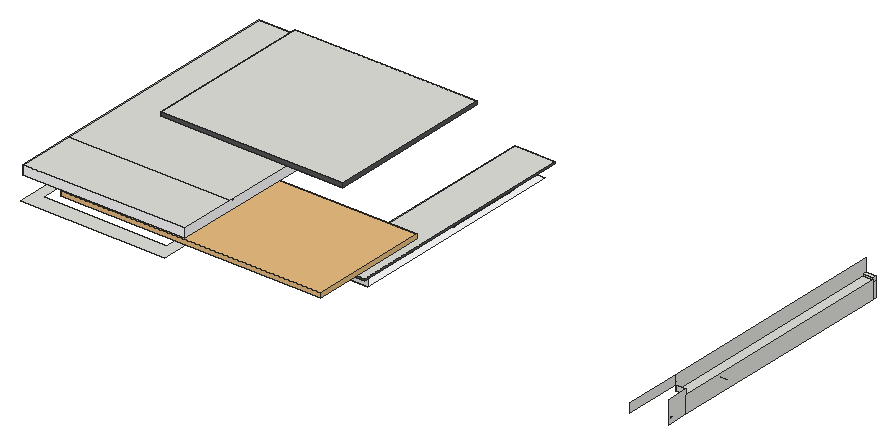
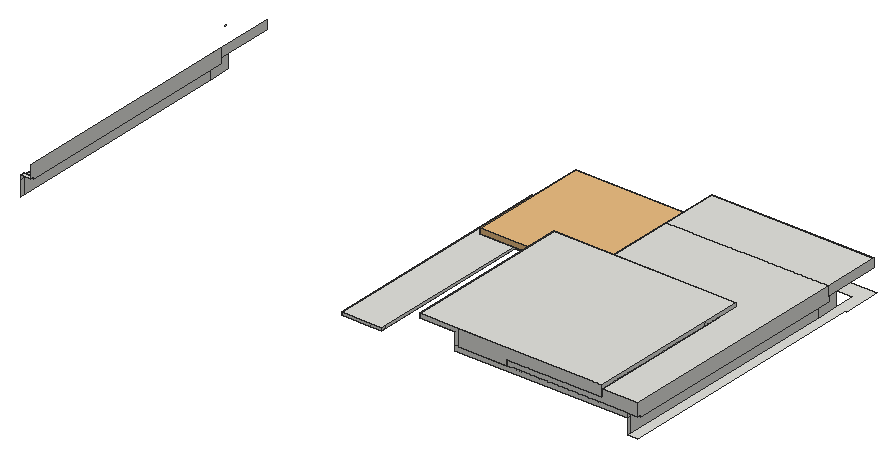
# SketchUp Ruby script. Lengths in inches.
U = 1.inch
M = Sketchup.active_model
def pt(a) = Geom::Point3d.new(a.map { |v| v * U })
def face(e, loops, mat)
  f = e.add_face(loops[0].map { |a| pt(a) })
  loops[1..].each { |l| e.add_face(l.map { |a| pt(a) }).erase! }
  f.material = f.back_material = mat if mat
  f
end
# faces: each face lists its corners as indices into pts; further lists are holes
def faces(e, pts, list, mat = nil) = list.each { |f| face(e, (f[0].is_a?(Array) ? f : [f]).map { |l| l.map { |i| pts[i] } }, mat) }
# xy, xz, yz: faces in a plane at the given z, y or x. An outline is a flat list of corners, or four numbers for a rectangle; further outlines are holes
def ring(l) = l.size == 4 ? [[l[0], l[1]], [l[2], l[1]], [l[2], l[3]], [l[0], l[3]]] : l.each_slice(2).to_a
def flat(e, list, mat, &to3) = list.each { |f| face(e, (f[0].is_a?(Array) ? f : [f]).map { |l| ring(l).map { |u, v| to3.(u, v) } }, mat) }
def xy(e, z, list, mat = nil) = flat(e, list, mat) { |x, y| [x, y, z] }
def xz(e, y, list, mat = nil) = flat(e, list, mat) { |x, z| [x, y, z] }
def yz(e, x, list, mat = nil) = flat(e, list, mat) { |y, z| [x, y, z] }
def lines(e, pts, list) = list.each { |a, b| e.add_line(pt(pts[a]), pt(pts[b])) }
# prism: a flat outline (further loops are holes) pulled along v
def prism(e, loops, v, mat = nil)
  f = face(e, loops, mat); d = Geom::Vector3d.new(v.map { |x| x * U })
  f.pushpull(f.normal.samedirection?(d) ? d.length : -d.length)
end
def box(e, o, s, mat = nil) = prism(e, [[o, [o[0] + s[0], o[1], o[2]], [o[0] + s[0], o[1] + s[1], o[2]], [o[0], o[1] + s[1], o[2]]]], [0, 0, s[2]], mat)
def at(x, y, z, deg = 0) = Geom::Transformation.translation(pt([x, y, z])) * Geom::Transformation.rotation(ORIGIN, Z_AXIS, deg.degrees)
def axes(o, x, y, z) = Geom::Transformation.new([*x, 0, *y, 0, *z, 0, *pt(o).to_a, 1])
def part(name) = M.definitions.add(name)
# library, detail: a bought-in or finely detailed component or shape, given as its bounding box
def library(name, o, s) = part(name).tap { |d| box(d.entities, o, s) }
def detail(e, o, s) = box(e.add_group.entities, o, s)
def put(e, d, t, mat = nil) = e.add_instance(d, t).tap { |i| i.material = mat if mat }
def group(e, t, mat = nil) = e.add_group.tap { |g| g.transformation = t; g.material = mat if mat }.entities
root = M.entities
M.materials.add("[Color M00]").color = [255, 255, 255]
M.materials.add("[Color M06]").color = [86, 86, 86]
c1 = library("Mesh Light\#4",[-0.5,-0.5,-0.1],[1,1,0.2])
c2 = part("Group\#24")
xy(c2.entities,0,[[203.13,95.41,201.58,95.62,200.13,96.22,198.89,97.17,197.9375,98.41,197.34,99.86,197.13,101.41,197.34,102.96,197.9375,104.41,198.89,105.65,200.13,106.61,201.58,107.21,203.13,107.41,204.6875,107.21,206.13,106.61,207.375,105.65,208.33,104.41,208.93,102.96,209.13,101.41,208.93,99.86,208.33,98.41,207.375,97.17,206.13,96.22,204.6875,95.62],[281.57,95.41,280.02,95.62,278.57,96.22,277.33,97.17,276.375,98.41,275.77,99.86,275.57,101.41,275.77,102.96,276.375,104.41,277.33,105.65,278.57,106.61,280.02,107.21,281.57,107.41,283.125,107.21,284.57,106.61,285.8125,105.65,286.77,104.41,287.37,102.96,287.57,101.41,287.37,99.86,286.77,98.41,285.8125,97.17,284.57,96.22,283.125,95.62],[350.95,95.41,349.39,95.62,347.95,96.22,346.7,97.17,345.75,98.41,345.15,99.86,344.95,101.41,345.15,102.96,345.75,104.41,346.7,105.65,347.95,106.61,349.39,107.21,350.95,107.41,352.5,107.21,353.95,106.61,355.1875,105.65,356.14,104.41,356.74,102.96,356.95,101.41,356.74,99.86,356.14,98.41,355.1875,97.17,353.95,96.22,352.5,95.62],[376,162.85,374.44,163.05,373,163.65,371.75,164.6,370.8,165.85,370.2,167.29,370,168.85,370.2,170.4,370.8,171.85,371.75,173.09,373,174.04,374.44,174.64,376,174.85,377.55,174.64,379,174.04,380.24,173.09,381.19,171.85,381.79,170.4,382,168.85,381.79,167.29,381.19,165.85,380.24,164.6,379,163.65,377.55,163.05]],"[Color M00]")
xy(c2.entities,33.4375,[[6,0,4.45,0.2,3,0.8,1.76,1.76,0.8,3,0.2,4.45,0,6,0.2,7.55,0.8,9,1.76,10.24,3,11.2,4.45,11.8,6,12,7.55,11.8,9,11.2,10.24,10.24,11.2,9,11.8,7.55,12,6,11.8,4.45,11.2,3,10.24,1.76,9,0.8,7.55,0.2],[83.125,0,81.57,0.2,80.125,0.8,78.88,1.76,77.93,3,77.33,4.45,77.125,6,77.33,7.55,77.93,9,78.88,10.24,80.125,11.2,81.57,11.8,83.125,12,84.68,11.8,86.125,11.2,87.37,10.24,88.32,9,88.92,7.55,89.125,6,88.92,4.45,88.32,3,87.37,1.76,86.125,0.8,84.68,0.2],[166.6875,0,165.13,0.2,163.6875,0.8,162.44,1.76,161.49,3,160.89,4.45,160.6875,6,160.89,7.55,161.49,9,162.44,10.24,163.6875,11.2,165.13,11.8,166.6875,12,168.24,11.8,169.6875,11.2,170.93,10.24,171.88,9,172.48,7.55,172.6875,6,172.48,4.45,171.88,3,170.93,1.76,169.6875,0.8,168.24,0.2],[166.6875,88.9375,165.13,89.14,163.6875,89.74,162.44,90.69,161.49,91.9375,160.89,93.38,160.6875,94.9375,160.89,96.49,161.49,97.9375,162.44,99.18,163.6875,100.13,165.13,100.73,166.6875,100.9375,168.24,100.73,169.6875,100.13,170.93,99.18,171.88,97.9375,172.48,96.49,172.6875,94.9375,172.48,93.38,171.88,91.9375,170.93,90.69,169.6875,89.74,168.24,89.14]],"[Color M00]")
put(c2.entities,c1,axes([191,87.42,16.72],[382.99758,0,0],[0,175.84579,0],[0,0,34.4375]))
c3 = library("Group\#23",[-0.5,-0.5,-0.1],[13,110.375,0.2])
xy(root,269.375,[[278.36,584.06,490.8,584.06,490.8,676.67,484.3,676.67,484.3,706.17,475.29,706.17,475.29,607.33,294.47,607.33,294.47,1021.31,279.74,1021.31,279.74,638.99,278.36,638.99],[484.3,676.67,490.8,731.24]])
xy(root,269.375,[[[490.8,676.67,490.8,731.24,674.49,731.24,674.49,1001.66,715.11,1001.66,715.11,676.67],[604.45,698.72,606.01,698.92,607.45,699.52,608.7,700.47,609.65,701.72,610.25,703.16,610.45,704.72,610.25,706.27,609.65,707.72,608.7,708.96,607.45,709.91,606.01,710.51,604.45,710.72,602.9,710.51,601.45,709.91,600.21,708.96,599.26,707.72,598.66,706.27,598.45,704.72,598.66,703.16,599.26,701.72,600.21,700.47,601.45,699.52,602.9,698.92],[673.83,698.72,675.38,698.92,676.83,699.52,678.07,700.47,679.02,701.72,679.625,703.16,679.83,704.72,679.625,706.27,679.02,707.72,678.07,708.96,676.83,709.91,675.38,710.51,673.83,710.72,672.27,710.51,670.83,709.91,669.59,708.96,668.63,707.72,668.03,706.27,667.83,704.72,668.03,703.16,668.63,701.72,669.59,700.47,670.83,699.52,672.27,698.92],[526.02,698.72,527.57,698.92,529.02,699.52,530.26,700.47,531.21,701.72,531.8125,703.16,532.02,704.72,531.8125,706.27,531.21,707.72,530.26,708.96,529.02,709.91,527.57,710.51,526.02,710.72,524.46,710.51,523.02,709.91,521.77,708.96,520.82,707.72,520.22,706.27,520.02,704.72,520.22,703.16,520.82,701.72,521.77,700.47,523.02,699.52,524.46,698.92],[698.88,766.15,700.43,766.35,701.88,766.95,703.12,767.91,704.08,769.15,704.68,770.6,704.88,772.15,704.68,773.7,704.08,775.15,703.12,776.39,701.88,777.35,700.43,777.95,698.88,778.15,697.33,777.95,695.88,777.35,694.64,776.39,693.68,775.15,693.08,773.7,692.88,772.15,693.08,770.6,693.68,769.15,694.64,767.91,695.88,766.95,697.33,766.35],[698.88,846.59,700.43,846.79,701.88,847.39,703.12,848.35,704.08,849.59,704.68,851.04,704.88,852.59,704.68,854.14,704.08,855.59,703.12,856.83,701.88,857.78,700.43,858.38,698.88,858.59,697.33,858.38,695.88,857.78,694.64,856.83,693.68,855.59,693.08,854.14,692.88,852.59,693.08,851.04,693.68,849.59,694.64,848.35,695.88,847.39,697.33,846.79],[698.88,943.96,700.43,944.17,701.88,944.77,703.12,945.72,704.08,946.96,704.68,948.41,704.88,949.96,704.68,951.52,704.08,952.96,703.12,954.21,701.88,955.16,700.43,955.76,698.88,955.96,697.33,955.76,695.88,955.16,694.64,954.21,693.68,952.96,693.08,951.52,692.88,949.96,693.08,948.41,693.68,946.96,694.64,945.72,695.88,944.77,697.33,944.17]]],"[Color M00]")
xy(root,279.25,[[484.3,670.42,715.11,676.67],[484.3,676.67,484.3,776.62,655.66,776.62,655.66,1021.31,715.11,1021.31,715.11,676.67]])
xy(root,282.6875,[[484.3,670.42,715.11,670.42,715.11,1021.31,655.66,1021.31,655.66,776.62,484.3,776.62]])
xy(root,291.125,[[304.78,733.75,304.78,1014.93,471.68,1014.93,471.68,854.49,462.15,854.49,462.15,733.75],[471.68,854.49,542.11,1014.93]])
xy(root,294.9375,[[279.74,670.48,294.47,1014.93],[1172.33,670.48,1187.0625,1014.93]])
xy(root,297.875,[[279.74,1014.93,294.47,1021.31],[294.47,1014.93,471.68,1021.31],[471.68,1014.93,542.11,1021.31],[1172.33,1014.93,1187.0625,1021.31]])
xy(root,302.8125,[[[279.74,587.17,279.74,670.48,294.47,670.48,294.47,639.17,471.68,639.17,471.68,832.12,518.11,832.12,518.11,587.17],[328.88,603.3,330.44,603.51,331.88,604.11,333.125,605.0625,334.08,606.3,334.68,607.75,334.88,609.3,334.68,610.86,334.08,612.3,333.125,613.55,331.88,614.5,330.44,615.1,328.88,615.3,327.33,615.1,325.88,614.5,324.64,613.55,323.6875,612.3,323.09,610.86,322.88,609.3,323.09,607.75,323.6875,606.3,324.64,605.0625,325.88,604.11,327.33,603.51],[406.01,603.3,407.56,603.51,409.01,604.11,410.25,605.0625,411.2,606.3,411.8,607.75,412.01,609.3,411.8,610.86,411.2,612.3,410.25,613.55,409.01,614.5,407.56,615.1,406.01,615.3,404.45,615.1,403.01,614.5,401.76,613.55,400.8125,612.3,400.21,610.86,400.01,609.3,400.21,607.75,400.8125,606.3,401.76,605.0625,403.01,604.11,404.45,603.51],[489.57,692.24,491.12,692.45,492.57,693.05,493.8125,694,494.77,695.24,495.37,696.6875,495.57,698.24,495.37,699.8,494.77,701.24,493.8125,702.48,492.57,703.4375,491.12,704.04,489.57,704.24,488.02,704.04,486.57,703.4375,485.33,702.48,484.375,701.24,483.77,699.8,483.57,698.24,483.77,696.6875,484.375,695.24,485.33,694,486.57,693.05,488.02,692.45],[489.57,603.3,491.12,603.51,492.57,604.11,493.8125,605.0625,494.77,606.3,495.37,607.75,495.57,609.3,495.37,610.86,494.77,612.3,493.8125,613.55,492.57,614.5,491.12,615.1,489.57,615.3,488.02,615.1,486.57,614.5,485.33,613.55,484.375,612.3,483.77,610.86,483.57,609.3,483.77,607.75,484.375,606.3,485.33,605.0625,486.57,604.11,488.02,603.51]]],"[Color M00]")
xy(root,305.625,[[332.11,832.12,471.68,1021.31]])
xy(root,316.0625,[[279.74,587.17,518.11,670.48],[279.74,670.48,518.11,670.48,518.11,774.49,332.11,774.49,332.11,1021.31,279.74,1021.31],[518.11,774.49,518.11,832.12,548.11,832.12,548.11,1021.31,599.68,1021.31,599.68,774.49]])
xy(root,321.8125,[[332.11,774.49,599.68,1021.31]])
xz(root,587.17,[[279.74,302.8125,518.11,316.0625]],"[Color M00]")
xz(root,670.42,[[484.3,279.25,715.11,282.6875]],"[Color M06]")
xz(root,670.48,[[279.74,294.9375,294.47,302.8125],[1172.33,294.9375,1187.0625,302.8125]])
xz(root,676.67,[[484.3,269.375,715.11,279.25]])
xz(root,774.49,[[332.11,316.0625,599.68,321.8125]],"[Color M06]")
xz(root,776.62,[[484.3,279.25,655.66,282.6875]])
xz(root,832.12,[[471.68,302.8125,518.11,305.625]])
xz(root,1014.93,[[294.47,291.125,471.68,297.875],[471.68,291.125,542.11,297.875],[279.74,294.9375,294.47,297.875],[1172.33,294.9375,1187.0625,297.875]])
xz(root,1021.31,[[655.66,279.25,671.36,282.6875],[671.36,279.25,715.11,282.6875],[294.47,291.125,548.11,297.875],[279.74,297.875,279.74,316.0625,332.11,316.0625,332.11,305.625,471.68,305.625,471.68,297.875],[471.68,297.875,471.68,305.625,332.11,305.625,332.11,321.8125,542.11,321.8125,542.11,297.875],
  [542.11,297.875,542.11,321.8125,599.68,321.8125,599.68,316.0625,548.11,316.0625,548.11,297.875]])
yz(root,279.74,[[670.48,294.9375,670.48,316.0625,1021.31,316.0625,1021.31,297.875,1014.93,297.875,1014.93,294.9375],[587.17,302.8125,670.48,316.0625]])
yz(root,294.47,[[639.17,269.375,670.48,302.8125],[670.48,269.375,1014.93,294.9375],[1014.93,269.375,1021.31,291.125],[1014.93,291.125,1021.31,297.875]])
yz(root,332.11,[[804.12,305.625,832.12,316.0625],[832.12,305.625,1021.31,316.0625],[774.49,316.0625,832.12,321.8125],[832.12,316.0625,1021.31,321.8125]])
yz(root,471.68,[[832.12,291.125,1014.93,297.875],[832.12,297.875,1021.31,305.625]])
yz(root,484.3,[[670.42,279.25,776.62,282.6875]])
yz(root,518.11,[[587.17,302.8125,832.12,316.0625]],"[Color M00]")
yz(root,599.68,[[774.49,316.0625,1021.31,321.8125]],"[Color M06]")
yz(root,655.66,[[776.62,279.25,1014.93,282.6875],[1014.93,279.25,1021.31,282.6875]])
yz(root,715.11,[[670.42,279.25,1021.31,282.6875]],"[Color M06]")
yz(root,1172.33,[[670.48,294.9375,670.48,316.0625,1021.31,316.0625,1021.31,297.875,1014.93,297.875,1014.93,294.9375],[587.17,302.8125,670.48,316.0625]])
yz(root,1187.0625,[[639.17,269.375,670.48,302.8125],[670.48,269.375,1014.93,294.9375],[1014.93,269.375,1021.31,291.125],[1014.93,291.125,1021.31,297.875]])
p = [[526.02,698.72,269.375],[524.46,698.92,269.375],[524.46,698.92,270.0625],[526.02,698.72,270.0625],[527.57,698.92,269.375],[527.57,698.92,270.0625],
  [604.45,698.72,269.375],[602.9,698.92,269.375],[602.9,698.92,270.0625],[604.45,698.72,270.0625],[606.01,698.92,269.375],[606.01,698.92,270.0625],
  [673.83,698.72,269.375],[672.27,698.92,269.375],[672.27,698.92,270.0625],[673.83,698.72,270.0625],[675.38,698.92,269.375],[675.38,698.92,270.0625],
  [523.02,699.52,269.375],[523.02,699.52,270.0625],[529.02,699.52,269.375],[529.02,699.52,270.0625],[601.45,699.52,269.375],[601.45,699.52,270.0625],
  [607.45,699.52,269.375],[607.45,699.52,270.0625],[670.83,699.52,269.375],[670.83,699.52,270.0625],[676.83,699.52,269.375],[676.83,699.52,270.0625],
  [521.77,700.47,269.375],[521.77,700.47,270.0625],[530.26,700.47,269.375],[530.26,700.47,270.0625],[600.21,700.47,269.375],[600.21,700.47,270.0625],
  [608.7,700.47,269.375],[608.7,700.47,270.0625],[669.59,700.47,269.375],[669.59,700.47,270.0625],[678.07,700.47,269.375],[678.07,700.47,270.0625],
  [520.82,701.72,269.375],[520.82,701.72,270.0625],[531.21,701.72,269.375],[531.21,701.72,270.0625],[599.26,701.72,269.375],[599.26,701.72,270.0625],
  [609.65,701.72,269.375],[609.65,701.72,270.0625],[668.63,701.72,269.375],[668.63,701.72,270.0625],[679.02,701.72,269.375],[679.02,701.72,270.0625],
  [520.22,703.16,269.375],[520.22,703.16,270.0625],[531.8125,703.16,269.375],[531.8125,703.16,270.0625],[598.66,703.16,269.375],[598.66,703.16,270.0625],
  [610.25,703.16,269.375],[610.25,703.16,270.0625],[668.03,703.16,269.375],[668.03,703.16,270.0625],[679.625,703.16,269.375],[679.625,703.16,270.0625],
  [520.02,704.72,269.375],[520.02,704.72,270.0625],[532.02,704.72,269.375],[532.02,704.72,270.0625],[598.45,704.72,269.375],[598.45,704.72,270.0625],
  [610.45,704.72,269.375],[610.45,704.72,270.0625],[667.83,704.72,269.375],[667.83,704.72,270.0625],[679.83,704.72,269.375],[679.83,704.72,270.0625],
  [520.22,706.27,269.375],[520.22,706.27,270.0625],[531.8125,706.27,269.375],[531.8125,706.27,270.0625],[598.66,706.27,269.375],[598.66,706.27,270.0625],
  [610.25,706.27,269.375],[610.25,706.27,270.0625],[668.03,706.27,269.375],[668.03,706.27,270.0625],[679.625,706.27,269.375],[679.625,706.27,270.0625],
  [520.82,707.72,269.375],[520.82,707.72,270.0625],[531.21,707.72,269.375],[531.21,707.72,270.0625],[599.26,707.72,269.375],[599.26,707.72,270.0625],
  [609.65,707.72,269.375],[609.65,707.72,270.0625],[668.63,707.72,269.375],[668.63,707.72,270.0625],[679.02,707.72,269.375],[679.02,707.72,270.0625],
  [521.77,708.96,269.375],[521.77,708.96,270.0625],[530.26,708.96,269.375],[530.26,708.96,270.0625],[600.21,708.96,269.375],[600.21,708.96,270.0625],
  [608.7,708.96,269.375],[608.7,708.96,270.0625],[669.59,708.96,269.375],[669.59,708.96,270.0625],[678.07,708.96,269.375],[678.07,708.96,270.0625],
  [523.02,709.91,269.375],[523.02,709.91,270.0625],[529.02,709.91,269.375],[529.02,709.91,270.0625],[601.45,709.91,269.375],[601.45,709.91,270.0625],
  [607.45,709.91,269.375],[607.45,709.91,270.0625],[670.83,709.91,269.375],[670.83,709.91,270.0625],[676.83,709.91,269.375],[676.83,709.91,270.0625],
  [524.46,710.51,269.375],[524.46,710.51,270.0625],[527.57,710.51,269.375],[527.57,710.51,270.0625],[602.9,710.51,269.375],[602.9,710.51,270.0625],
  [606.01,710.51,269.375],[606.01,710.51,270.0625],[672.27,710.51,269.375],[672.27,710.51,270.0625],[675.38,710.51,269.375],[675.38,710.51,270.0625],
  [526.02,710.72,269.375],[526.02,710.72,270.0625],[604.45,710.72,269.375],[604.45,710.72,270.0625],[673.83,710.72,269.375],[673.83,710.72,270.0625],
  [698.88,766.15,269.375],[697.33,766.35,269.375],[697.33,766.35,270.0625],[698.88,766.15,270.0625],[700.43,766.35,269.375],[700.43,766.35,270.0625],
  [695.88,766.95,269.375],[695.88,766.95,270.0625],[701.88,766.95,269.375],[701.88,766.95,270.0625],[694.64,767.91,269.375],[694.64,767.91,270.0625],
  [703.12,767.91,269.375],[703.12,767.91,270.0625],[693.68,769.15,269.375],[693.68,769.15,270.0625],[704.08,769.15,269.375],[704.08,769.15,270.0625],
  [693.08,770.6,269.375],[693.08,770.6,270.0625],[704.68,770.6,269.375],[704.68,770.6,270.0625],[692.88,772.15,269.375],[692.88,772.15,270.0625],
  [704.88,772.15,269.375],[704.88,772.15,270.0625],[693.08,773.7,269.375],[693.08,773.7,270.0625],[704.68,773.7,269.375],[704.68,773.7,270.0625],
  [693.68,775.15,269.375],[693.68,775.15,270.0625],[704.08,775.15,269.375],[704.08,775.15,270.0625],[694.64,776.39,269.375],[694.64,776.39,270.0625],
  [703.12,776.39,269.375],[703.12,776.39,270.0625],[695.88,777.35,269.375],[695.88,777.35,270.0625],[701.88,777.35,269.375],[701.88,777.35,270.0625],
  [697.33,777.95,269.375],[697.33,777.95,270.0625],[700.43,777.95,269.375],[700.43,777.95,270.0625],[698.88,778.15,269.375],[698.88,778.15,270.0625],
  [698.88,846.59,269.375],[697.33,846.79,269.375],[697.33,846.79,270.0625],[698.88,846.59,270.0625],[700.43,846.79,269.375],[700.43,846.79,270.0625],
  [695.88,847.39,269.375],[695.88,847.39,270.0625],[701.88,847.39,269.375],[701.88,847.39,270.0625],[694.64,848.35,269.375],[694.64,848.35,270.0625],
  [703.12,848.35,269.375],[703.12,848.35,270.0625],[693.68,849.59,269.375],[693.68,849.59,270.0625],[704.08,849.59,269.375],[704.08,849.59,270.0625],
  [693.08,851.04,269.375],[693.08,851.04,270.0625],[704.68,851.04,269.375],[704.68,851.04,270.0625],[692.88,852.59,269.375],[692.88,852.59,270.0625],
  [704.88,852.59,269.375],[704.88,852.59,270.0625],[693.08,854.14,269.375],[693.08,854.14,270.0625],[704.68,854.14,269.375],[704.68,854.14,270.0625],
  [693.68,855.59,269.375],[693.68,855.59,270.0625],[704.08,855.59,269.375],[704.08,855.59,270.0625],[694.64,856.83,269.375],[694.64,856.83,270.0625],
  [703.12,856.83,269.375],[703.12,856.83,270.0625],[695.88,857.78,269.375],[695.88,857.78,270.0625],[701.88,857.78,269.375],[701.88,857.78,270.0625],
  [697.33,858.38,269.375],[697.33,858.38,270.0625],[700.43,858.38,269.375],[700.43,858.38,270.0625],[698.88,858.59,269.375],[698.88,858.59,270.0625],
  [698.88,943.96,269.375],[697.33,944.17,269.375],[697.33,944.17,270.0625],[698.88,943.96,270.0625],[700.43,944.17,269.375],[700.43,944.17,270.0625],
  [695.88,944.77,269.375],[695.88,944.77,270.0625],[701.88,944.77,269.375],[701.88,944.77,270.0625],[694.64,945.72,269.375],[694.64,945.72,270.0625],
  [703.12,945.72,269.375],[703.12,945.72,270.0625],[693.68,946.96,269.375],[693.68,946.96,270.0625],[704.08,946.96,269.375],[704.08,946.96,270.0625],
  [693.08,948.41,269.375],[693.08,948.41,270.0625],[704.68,948.41,269.375],[704.68,948.41,270.0625],[692.88,949.96,269.375],[692.88,949.96,270.0625],
  [704.88,949.96,269.375],[704.88,949.96,270.0625],[693.08,951.52,269.375],[693.08,951.52,270.0625],[704.68,951.52,269.375],[704.68,951.52,270.0625],
  [693.68,952.96,269.375],[693.68,952.96,270.0625],[704.08,952.96,269.375],[704.08,952.96,270.0625],[694.64,954.21,269.375],[694.64,954.21,270.0625],
  [703.12,954.21,269.375],[703.12,954.21,270.0625],[695.88,955.16,269.375],[695.88,955.16,270.0625],[701.88,955.16,269.375],[701.88,955.16,270.0625],
  [697.33,955.76,269.375],[697.33,955.76,270.0625],[700.43,955.76,269.375],[700.43,955.76,270.0625],[698.88,955.96,269.375],[698.88,955.96,270.0625],
  [328.88,603.3,302.8125],[327.33,603.51,302.8125],[327.33,603.51,303.5],[328.88,603.3,303.5],[330.44,603.51,302.8125],[330.44,603.51,303.5],
  [406.01,603.3,302.8125],[404.45,603.51,302.8125],[404.45,603.51,303.5],[406.01,603.3,303.5],[407.56,603.51,302.8125],[407.56,603.51,303.5],
  [489.57,603.3,302.8125],[488.02,603.51,302.8125],[488.02,603.51,303.5],[489.57,603.3,303.5],[491.12,603.51,302.8125],[491.12,603.51,303.5],
  [325.88,604.11,302.8125],[325.88,604.11,303.5],[331.88,604.11,302.8125],[331.88,604.11,303.5],[403.01,604.11,302.8125],[403.01,604.11,303.5],
  [409.01,604.11,302.8125],[409.01,604.11,303.5],[486.57,604.11,302.8125],[486.57,604.11,303.5],[492.57,604.11,302.8125],[492.57,604.11,303.5],
  [324.64,605.0625,302.8125],[324.64,605.0625,303.5],[333.125,605.0625,302.8125],[333.125,605.0625,303.5],[401.76,605.0625,302.8125],[401.76,605.0625,303.5],
  [410.25,605.0625,302.8125],[410.25,605.0625,303.5],[485.33,605.0625,302.8125],[485.33,605.0625,303.5],[493.8125,605.0625,302.8125],[493.8125,605.0625,303.5],
  [323.6875,606.3,302.8125],[323.6875,606.3,303.5],[334.08,606.3,302.8125],[334.08,606.3,303.5],[400.8125,606.3,302.8125],[400.8125,606.3,303.5],
  [411.2,606.3,302.8125],[411.2,606.3,303.5],[484.375,606.3,302.8125],[484.375,606.3,303.5],[494.77,606.3,302.8125],[494.77,606.3,303.5],
  [323.09,607.75,302.8125],[323.09,607.75,303.5],[334.68,607.75,302.8125],[334.68,607.75,303.5],[400.21,607.75,302.8125],[400.21,607.75,303.5],
  [411.8,607.75,302.8125],[411.8,607.75,303.5],[483.77,607.75,302.8125],[483.77,607.75,303.5],[495.37,607.75,302.8125],[495.37,607.75,303.5],
  [322.88,609.3,302.8125],[322.88,609.3,303.5],[334.88,609.3,302.8125],[334.88,609.3,303.5],[400.01,609.3,302.8125],[400.01,609.3,303.5],
  [412.01,609.3,302.8125],[412.01,609.3,303.5],[483.57,609.3,302.8125],[483.57,609.3,303.5],[495.57,609.3,302.8125],[495.57,609.3,303.5],
  [1215.68,607.75,302.8125],[1215.47,609.3,302.8125],[1215.47,609.3,303.5],[1215.68,607.75,303.5],[323.09,610.86,302.8125],[323.09,610.86,303.5],
  [334.68,610.86,302.8125],[334.68,610.86,303.5],[400.21,610.86,302.8125],[400.21,610.86,303.5],[411.8,610.86,302.8125],[411.8,610.86,303.5],
  [483.77,610.86,302.8125],[483.77,610.86,303.5],[495.37,610.86,302.8125],[495.37,610.86,303.5],[323.6875,612.3,302.8125],[323.6875,612.3,303.5],
  [334.08,612.3,302.8125],[334.08,612.3,303.5],[400.8125,612.3,302.8125],[400.8125,612.3,303.5],[411.2,612.3,302.8125],[411.2,612.3,303.5],
  [484.375,612.3,302.8125],[484.375,612.3,303.5],[494.77,612.3,302.8125],[494.77,612.3,303.5],[324.64,613.55,302.8125],[324.64,613.55,303.5],
  [333.125,613.55,302.8125],[333.125,613.55,303.5],[401.76,613.55,302.8125],[401.76,613.55,303.5],[410.25,613.55,302.8125],[410.25,613.55,303.5],
  [485.33,613.55,302.8125],[485.33,613.55,303.5],[493.8125,613.55,302.8125],[493.8125,613.55,303.5],[325.88,614.5,302.8125],[325.88,614.5,303.5],
  [331.88,614.5,302.8125],[331.88,614.5,303.5],[403.01,614.5,302.8125],[403.01,614.5,303.5],[409.01,614.5,302.8125],[409.01,614.5,303.5],
  [486.57,614.5,302.8125],[486.57,614.5,303.5],[492.57,614.5,302.8125],[492.57,614.5,303.5],[327.33,615.1,302.8125],[327.33,615.1,303.5],
  [330.44,615.1,302.8125],[330.44,615.1,303.5],[404.45,615.1,302.8125],[404.45,615.1,303.5],[407.56,615.1,302.8125],[407.56,615.1,303.5],
  [488.02,615.1,302.8125],[488.02,615.1,303.5],[491.12,615.1,302.8125],[491.12,615.1,303.5],[328.88,615.3,302.8125],[328.88,615.3,303.5],
  [406.01,615.3,302.8125],[406.01,615.3,303.5],[489.57,615.3,302.8125],[489.57,615.3,303.5],[489.57,692.24,302.8125],[488.02,692.45,302.8125],
  [488.02,692.45,303.5],[489.57,692.24,303.5],[491.12,692.45,302.8125],[491.12,692.45,303.5],[486.57,693.05,302.8125],[486.57,693.05,303.5],
  [492.57,693.05,302.8125],[492.57,693.05,303.5],[485.33,694,302.8125],[485.33,694,303.5],[493.8125,694,302.8125],[493.8125,694,303.5],
  [484.375,695.24,302.8125],[484.375,695.24,303.5],[494.77,695.24,302.8125],[494.77,695.24,303.5],[483.77,696.6875,302.8125],[483.77,696.6875,303.5],
  [495.37,696.6875,302.8125],[495.37,696.6875,303.5],[483.57,698.24,302.8125],[483.57,698.24,303.5],[495.57,698.24,302.8125],[495.57,698.24,303.5],
  [483.77,699.8,302.8125],[483.77,699.8,303.5],[495.37,699.8,302.8125],[495.37,699.8,303.5],[484.375,701.24,302.8125],[484.375,701.24,303.5],
  [494.77,701.24,302.8125],[494.77,701.24,303.5],[485.33,702.48,302.8125],[485.33,702.48,303.5],[493.8125,702.48,302.8125],[493.8125,702.48,303.5],
  [486.57,703.4375,302.8125],[486.57,703.4375,303.5],[492.57,703.4375,302.8125],[492.57,703.4375,303.5],[488.02,704.04,302.8125],[488.02,704.04,303.5],
  [491.12,704.04,302.8125],[491.12,704.04,303.5],[489.57,704.24,302.8125],[489.57,704.24,303.5],[332.11,804.12,305.625],[501.74,804.12,305.625],
  [542.11,1014.93,297.875],[542.11,832.12,297.875],[542.11,854.49,291.125],[548.11,854.49,291.125],[674.49,1001.66,269.375],[674.49,1001.66,277.5],
  [542.11,832.12,291.125],[304.78,733.75,291.125],[294.47,733.75,291.125],[1197.375,733.75,291.125],[1187.0625,733.75,291.125]]
faces(root,p,[[0,1,2,3],[4,0,3,5],[6,7,8,9],[10,6,9,11],[12,13,14,15],[16,12,15,17],[1,18,19,2],[20,4,5,21],
  [7,22,23,8],[24,10,11,25],[13,26,27,14],[28,16,17,29],[18,30,31,19],[32,20,21,33],[22,34,35,23],[36,24,25,37],
  [26,38,39,27],[40,28,29,41],[30,42,43,31],[44,32,33,45],[34,46,47,35],[48,36,37,49],[38,50,51,39],[52,40,41,53],
  [42,54,55,43],[56,44,45,57],[46,58,59,47],[60,48,49,61],[50,62,63,51],[64,52,53,65],[54,66,67,55],[68,56,57,69],
  [58,70,71,59],[72,60,61,73],[62,74,75,63],[76,64,65,77],[66,78,79,67],[80,68,69,81],[70,82,83,71],[84,72,73,85],
  [74,86,87,75],[88,76,77,89],[78,90,91,79],[92,80,81,93],[82,94,95,83],[96,84,85,97],[86,98,99,87],[100,88,89,101],
  [90,102,103,91],[104,92,93,105],[94,106,107,95],[108,96,97,109],[98,110,111,99],[112,100,101,113],[102,114,115,103],[116,104,105,117],
  [106,118,119,107],[120,108,109,121],[110,122,123,111],[124,112,113,125],[114,126,127,115],[128,116,117,129],[118,130,131,119],[132,120,121,133],
  [122,134,135,123],[136,124,125,137],[126,138,139,127],[138,128,129,139],[130,140,141,131],[140,132,133,141],[134,142,143,135],[142,136,137,143],
  [144,145,146,147],[148,144,147,149],[145,150,151,146],[152,148,149,153],[150,154,155,151],[156,152,153,157],[154,158,159,155],[160,156,157,161],
  [158,162,163,159],[164,160,161,165],[162,166,167,163],[168,164,165,169],[166,170,171,167],[172,168,169,173],[170,174,175,171],[176,172,173,177],
  [174,178,179,175],[180,176,177,181],[178,182,183,179],[184,180,181,185],[182,186,187,183],[188,184,185,189],[186,190,191,187],[190,188,189,191],
  [192,193,194,195],[196,192,195,197],[193,198,199,194],[200,196,197,201],[198,202,203,199],[204,200,201,205],[202,206,207,203],[208,204,205,209],
  [206,210,211,207],[212,208,209,213],[210,214,215,211],[216,212,213,217],[214,218,219,215],[220,216,217,221],[218,222,223,219],[224,220,221,225],
  [222,226,227,223],[228,224,225,229],[226,230,231,227],[232,228,229,233],[230,234,235,231],[236,232,233,237],[234,238,239,235],[238,236,237,239],
  [240,241,242,243],[244,240,243,245],[241,246,247,242],[248,244,245,249],[246,250,251,247],[252,248,249,253],[250,254,255,251],[256,252,253,257],
  [254,258,259,255],[260,256,257,261],[258,262,263,259],[264,260,261,265],[262,266,267,263],[268,264,265,269],[266,270,271,267],[272,268,269,273],
  [270,274,275,271],[276,272,273,277],[274,278,279,275],[280,276,277,281],[278,282,283,279],[284,280,281,285],[282,286,287,283],[286,284,285,287],
  [288,289,290,291],[292,288,291,293],[294,295,296,297],[298,294,297,299],[300,301,302,303],[304,300,303,305],[289,306,307,290],[308,292,293,309],
  [295,310,311,296],[312,298,299,313],[301,314,315,302],[316,304,305,317],[306,318,319,307],[320,308,309,321],[310,322,323,311],[324,312,313,325],
  [314,326,327,315],[328,316,317,329],[318,330,331,319],[332,320,321,333],[322,334,335,323],[336,324,325,337],[326,338,339,327],[340,328,329,341],
  [330,342,343,331],[344,332,333,345],[334,346,347,335],[348,336,337,349],[338,350,351,339],[352,340,341,353],[342,354,355,343],[356,344,345,357],
  [346,358,359,347],[360,348,349,361],[350,362,363,351],[364,352,353,365],[366,367,368,369],[354,370,371,355],[372,356,357,373],[358,374,375,359],
  [376,360,361,377],[362,378,379,363],[380,364,365,381],[370,382,383,371],[384,372,373,385],[374,386,387,375],[388,376,377,389],[378,390,391,379],
  [392,380,381,393],[382,394,395,383],[396,384,385,397],[386,398,399,387],[400,388,389,401],[390,402,403,391],[404,392,393,405],[394,406,407,395],
  [408,396,397,409],[398,410,411,399],[412,400,401,413],[402,414,415,403],[416,404,405,417],[406,418,419,407],[420,408,409,421],[410,422,423,411],
  [424,412,413,425],[414,426,427,415],[428,416,417,429],[418,430,431,419],[430,420,421,431],[422,432,433,423],[432,424,425,433],[426,434,435,427],
  [434,428,429,435],[436,437,438,439],[440,436,439,441],[437,442,443,438],[444,440,441,445],[442,446,447,443],[448,444,445,449],[446,450,451,447],
  [452,448,449,453],[450,454,455,451],[456,452,453,457],[454,458,459,455],[460,456,457,461],[458,462,463,459],[464,460,461,465],[462,466,467,463],
  [468,464,465,469],[466,470,471,467],[472,468,469,473],[470,474,475,471],[476,472,473,477],[474,478,479,475],[480,476,477,481],[478,482,483,479],
  [482,480,481,483]],"[Color M00]")
lines(root,p,[[484,485],[486,487],[488,489],[490,491],[488,492],[493,494],[495,496]])
put(root,c2,at(322.88,603.3,270.0625))
put(root,c3,at(692.88,846.59,270.0625))
